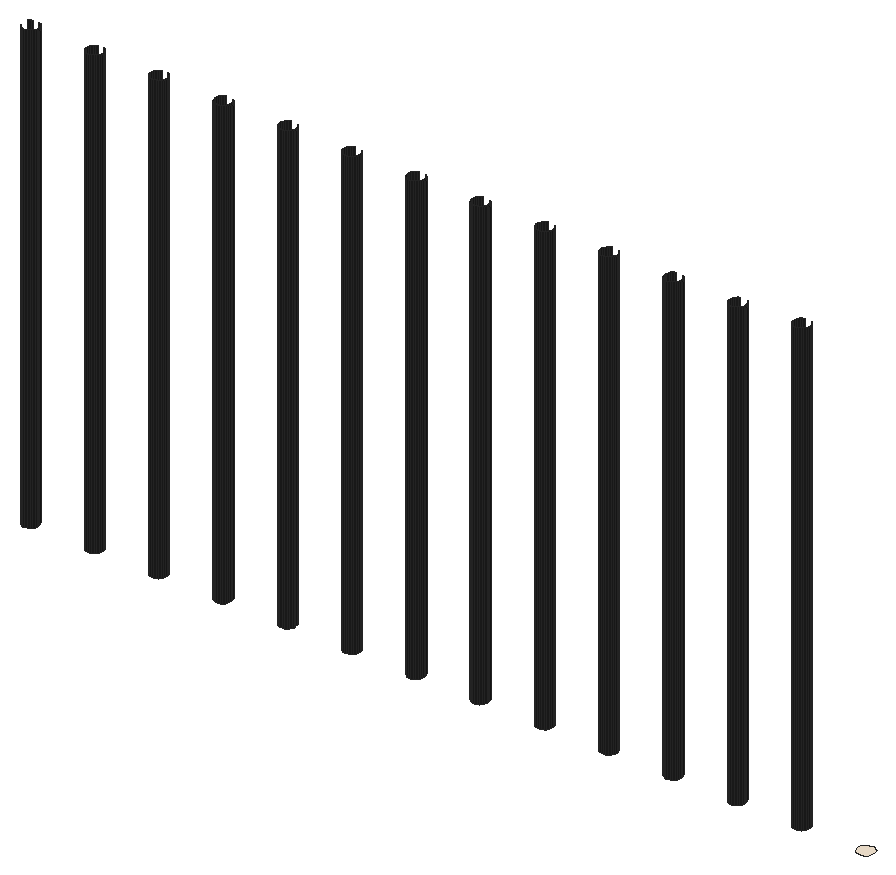
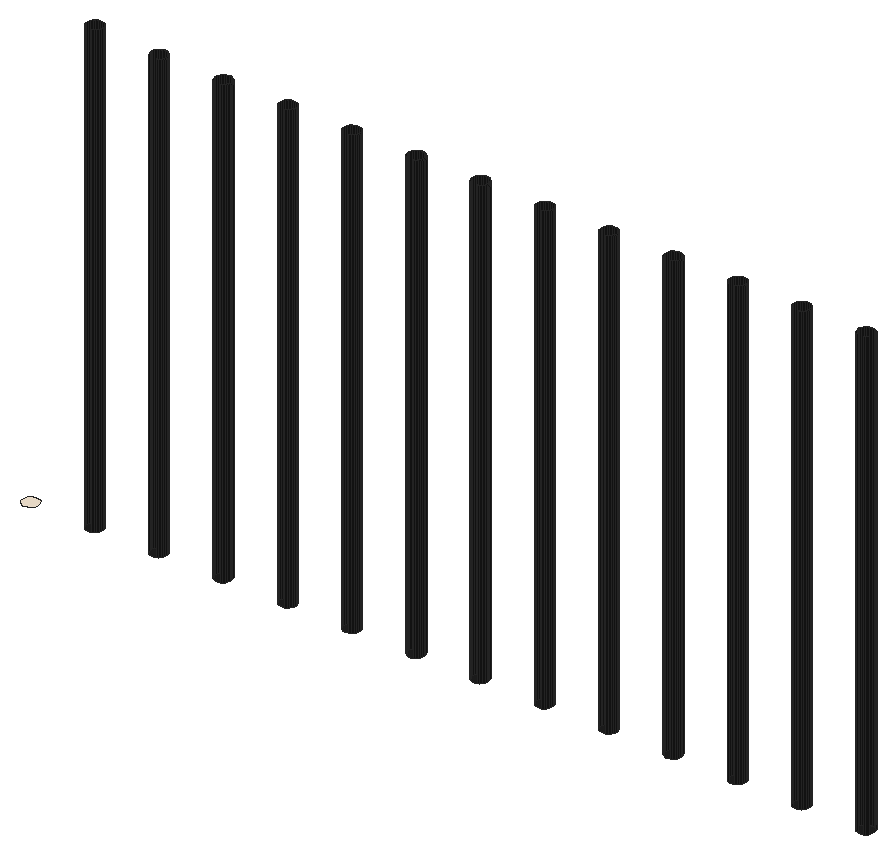
# SketchUp Ruby script. Lengths in inches.
U = 1.inch
M = Sketchup.active_model
def pt(a) = Geom::Point3d.new(a.map { |v| v * U })
def face(e, loops, mat)
  f = e.add_face(loops[0].map { |a| pt(a) })
  loops[1..].each { |l| e.add_face(l.map { |a| pt(a) }).erase! }
  f.material = f.back_material = mat if mat
  f
end
# faces: each face lists its corners as indices into pts; further lists are holes
def faces(e, pts, list, mat = nil) = list.each { |f| face(e, (f[0].is_a?(Array) ? f : [f]).map { |l| l.map { |i| pts[i] } }, mat) }
# xy, xz, yz: faces in a plane at the given z, y or x. An outline is a flat list of corners, or four numbers for a rectangle; further outlines are holes
def ring(l) = l.size == 4 ? [[l[0], l[1]], [l[2], l[1]], [l[2], l[3]], [l[0], l[3]]] : l.each_slice(2).to_a
def flat(e, list, mat, &to3) = list.each { |f| face(e, (f[0].is_a?(Array) ? f : [f]).map { |l| ring(l).map { |u, v| to3.(u, v) } }, mat) }
def xy(e, z, list, mat = nil) = flat(e, list, mat) { |x, y| [x, y, z] }
def xz(e, y, list, mat = nil) = flat(e, list, mat) { |x, z| [x, y, z] }
def yz(e, x, list, mat = nil) = flat(e, list, mat) { |y, z| [x, y, z] }
def lines(e, pts, list) = list.each { |a, b| e.add_line(pt(pts[a]), pt(pts[b])) }
# prism: a flat outline (further loops are holes) pulled along v
def prism(e, loops, v, mat = nil)
  f = face(e, loops, mat); d = Geom::Vector3d.new(v.map { |x| x * U })
  f.pushpull(f.normal.samedirection?(d) ? d.length : -d.length)
end
def box(e, o, s, mat = nil) = prism(e, [[o, [o[0] + s[0], o[1], o[2]], [o[0] + s[0], o[1] + s[1], o[2]], [o[0], o[1] + s[1], o[2]]]], [0, 0, s[2]], mat)
def at(x, y, z, deg = 0) = Geom::Transformation.translation(pt([x, y, z])) * Geom::Transformation.rotation(ORIGIN, Z_AXIS, deg.degrees)
def axes(o, x, y, z) = Geom::Transformation.new([*x, 0, *y, 0, *z, 0, *pt(o).to_a, 1])
def part(name) = M.definitions.add(name)
# library, detail: a bought-in or finely detailed component or shape, given as its bounding box
def library(name, o, s) = part(name).tap { |d| box(d.entities, o, s) }
def detail(e, o, s) = box(e.add_group.entities, o, s)
def put(e, d, t, mat = nil) = e.add_instance(d, t).tap { |i| i.material = mat if mat }
def group(e, t, mat = nil) = e.add_group.tap { |g| g.transformation = t; g.material = mat if mat }.entities
root = M.entities
M.materials.add("[0028_AntiqueWhite]").color = [250, 235, 215]
M.materials.add("[Color M08]").color = [30, 30, 30]
xy(root,177,[[209.92,194.68,210.0625,194.68,210.21,194.72,210.33,194.79,210.4375,194.89,210.51,195.02,210.55,195.16,210.55,195.31,210.51,195.45,210.44,195.58,210.33,195.68,210.2,195.75,210.0625,195.79,209.92,195.79,209.77,195.75,209.65,195.68,209.54,195.58,209.47,195.45,209.43,195.31,209.43,195.16,209.47,195.02,209.54,194.89,209.65,194.79,209.78,194.71]],"[0028_AntiqueWhite]")
xy(root,177,[[150.6,194.68,150.46,194.71,150.34,194.79,150.23,194.89,150.16,195.02,150.12,195.16,150.12,195.31,150.16,195.45,150.23,195.58,150.33,195.68,150.46,195.75,150.6,195.79,150.75,195.79,150.89,195.75,151.02,195.68,151.12,195.58,151.2,195.45,151.23,195.31,151.24,195.16,151.2,195.02,151.125,194.89,151.02,194.79,150.89,194.72,150.75,194.68],[155.17,194.68,155.03,194.71,154.9,194.79,154.79,194.89,154.72,195.02,154.68,195.16,154.68,195.31,154.72,195.45,154.79,195.58,154.9,195.68,155.02,195.75,155.17,195.79,155.3125,195.79,155.45,195.75,155.58,195.68,155.69,195.58,155.76,195.45,155.8,195.31,155.8,195.16,155.76,195.02,155.6875,194.89,155.58,194.79,155.46,194.72,155.3125,194.68],[159.73,194.68,159.59,194.71,159.46,194.79,159.36,194.89,159.28,195.02,159.24,195.16,159.24,195.31,159.28,195.45,159.36,195.58,159.46,195.68,159.59,195.75,159.73,195.79,159.875,195.79,160.02,195.75,160.14,195.68,160.25,195.58,160.32,195.45,160.36,195.31,160.36,195.16,160.32,195.02,160.25,194.89,160.15,194.79,160.02,194.72,159.875,194.68],[164.29,194.68,164.15,194.71,164.02,194.79,163.92,194.89,163.85,195.02,163.81,195.16,163.81,195.31,163.84,195.45,163.92,195.58,164.02,195.68,164.15,195.75,164.29,195.79,164.4375,195.79,164.58,195.75,164.71,195.68,164.81,195.58,164.88,195.45,164.92,195.31,164.92,195.16,164.88,195.02,164.8125,194.89,164.71,194.79,164.58,194.72,164.4375,194.68],[168.85,194.68,168.71,194.71,168.59,194.79,168.48,194.89,168.41,195.02,168.37,195.16,168.37,195.31,168.41,195.45,168.48,195.58,168.58,195.68,168.71,195.75,168.85,195.79,169,195.79,169.14,195.75,169.27,195.68,169.37,195.58,169.45,195.45,169.48,195.31,169.49,195.16,169.45,195.02,169.375,194.89,169.27,194.79,169.14,194.72,169,194.68],
  [173.42,194.68,173.28,194.71,173.15,194.79,173.04,194.89,172.97,195.02,172.93,195.16,172.93,195.31,172.97,195.45,173.04,195.58,173.15,195.68,173.27,195.75,173.42,195.79,173.5625,195.79,173.7,195.75,173.83,195.68,173.94,195.58,174.01,195.45,174.05,195.31,174.05,195.16,174.01,195.02,173.9375,194.89,173.83,194.79,173.71,194.72,173.5625,194.68],[177.98,194.68,177.84,194.71,177.71,194.79,177.61,194.89,177.53,195.02,177.49,195.16,177.49,195.31,177.53,195.45,177.61,195.58,177.71,195.68,177.84,195.75,177.98,195.79,178.125,195.79,178.27,195.75,178.39,195.68,178.5,195.58,178.57,195.45,178.61,195.31,178.61,195.16,178.57,195.02,178.5,194.89,178.4,194.79,178.27,194.72,178.125,194.68],[182.54,194.68,182.4,194.71,182.27,194.79,182.17,194.89,182.1,195.02,182.06,195.16,182.06,195.31,182.09,195.45,182.17,195.58,182.27,195.68,182.4,195.75,182.54,195.79,182.6875,195.79,182.83,195.75,182.96,195.68,183.06,195.58,183.13,195.45,183.17,195.31,183.17,195.16,183.13,195.02,183.0625,194.89,182.96,194.79,182.83,194.72,182.6875,194.68],[187.1,194.68,186.96,194.71,186.84,194.79,186.73,194.89,186.66,195.02,186.62,195.16,186.62,195.31,186.66,195.45,186.73,195.58,186.83,195.68,186.96,195.75,187.1,195.79,187.25,195.79,187.39,195.75,187.52,195.68,187.62,195.58,187.7,195.45,187.73,195.31,187.74,195.16,187.7,195.02,187.625,194.89,187.52,194.79,187.39,194.72,187.25,194.68],[191.67,194.68,191.53,194.71,191.4,194.79,191.29,194.89,191.22,195.02,191.18,195.16,191.18,195.31,191.22,195.45,191.29,195.58,191.4,195.68,191.52,195.75,191.67,195.79,191.8125,195.79,191.95,195.75,192.08,195.68,192.19,195.58,192.26,195.45,192.3,195.31,192.3,195.16,192.26,195.02,192.1875,194.89,192.08,194.79,191.96,194.72,191.8125,194.68],
  [196.23,194.68,196.09,194.71,195.96,194.79,195.86,194.89,195.78,195.02,195.74,195.16,195.74,195.31,195.78,195.45,195.86,195.58,195.96,195.68,196.09,195.75,196.23,195.79,196.375,195.79,196.52,195.75,196.64,195.68,196.75,195.58,196.82,195.45,196.86,195.31,196.86,195.16,196.82,195.02,196.75,194.89,196.65,194.79,196.52,194.72,196.375,194.68],[200.79,194.68,200.65,194.71,200.52,194.79,200.42,194.89,200.35,195.02,200.31,195.16,200.31,195.31,200.34,195.45,200.42,195.58,200.52,195.68,200.65,195.75,200.79,195.79,200.9375,195.79,201.08,195.75,201.21,195.68,201.31,195.58,201.38,195.45,201.42,195.31,201.42,195.16,201.38,195.02,201.3125,194.89,201.21,194.79,201.08,194.72,200.9375,194.68],[205.35,194.68,205.21,194.71,205.09,194.79,204.98,194.89,204.91,195.02,204.87,195.16,204.87,195.31,204.91,195.45,204.98,195.58,205.08,195.68,205.21,195.75,205.35,195.79,205.5,195.79,205.64,195.75,205.77,195.68,205.87,195.58,205.95,195.45,205.98,195.31,205.99,195.16,205.95,195.02,205.875,194.89,205.77,194.79,205.64,194.72,205.5,194.68]],"[Color M08]")
xz(root,194.68,[[150.6,177,150.75,208.66],[155.17,177,155.3125,208.66],[159.73,177,159.875,208.66],[164.29,177,164.4375,208.66],[168.85,177,169,208.66],
  [173.42,177,173.5625,208.625],[177.98,177,178.125,208.66],[182.54,177,182.6875,208.66],[187.1,177,187.25,208.66],[191.67,177,191.8125,208.66],
  [196.23,177,196.375,208.66],[200.79,177,200.9375,208.66],[205.35,177,205.5,208.9375]],"[Color M08]")
yz(root,154.68,[[195.16,177,195.31,208.66]],"[Color M08]")
yz(root,155.8,[[195.16,177,195.31,208.66]],"[Color M08]")
yz(root,159.24,[[195.16,177,195.31,208.66]],"[Color M08]")
yz(root,160.36,[[195.16,177,195.31,208.66]],"[Color M08]")
yz(root,163.81,[[195.16,177,195.31,208.66]],"[Color M08]")
yz(root,164.92,[[195.16,177,195.31,208.66]],"[Color M08]")
yz(root,168.37,[[195.16,177,195.31,208.66]],"[Color M08]")
yz(root,172.93,[[195.16,177,195.31,208.625]],"[Color M08]")
yz(root,174.05,[[195.16,177,195.31,208.625]],"[Color M08]")
yz(root,177.49,[[195.16,177,195.31,208.66]],"[Color M08]")
yz(root,178.61,[[195.16,177,195.31,208.66]],"[Color M08]")
yz(root,182.06,[[195.16,177,195.31,208.66]],"[Color M08]")
yz(root,183.17,[[195.16,177,195.31,208.66]],"[Color M08]")
yz(root,186.62,[[195.16,177,195.31,208.66]],"[Color M08]")
yz(root,191.18,[[195.16,177,195.31,208.66]],"[Color M08]")
yz(root,192.3,[[195.16,177,195.31,208.66]],"[Color M08]")
yz(root,195.74,[[195.16,177,195.31,208.66]],"[Color M08]")
yz(root,196.86,[[195.16,177,195.31,208.66]],"[Color M08]")
yz(root,200.31,[[195.16,177,195.31,208.66]],"[Color M08]")
yz(root,201.42,[[195.16,177,195.31,208.66]],"[Color M08]")
yz(root,204.87,[[195.16,177,195.31,208.9375]],"[Color M08]")
p = [[150.34,194.79,177],[150.46,194.71,177],[150.46,194.71,208.66],[150.34,194.79,208.66],[150.6,194.68,177],[150.6,194.68,208.66],
  [150.75,194.68,177],[150.89,194.72,177],[150.89,194.72,208.66],[150.75,194.68,208.66],[151.02,194.79,177],[151.02,194.79,208.66],
  [154.9,194.79,177],[155.03,194.71,177],[155.03,194.71,208.66],[154.9,194.79,208.66],[155.17,194.68,177],[155.17,194.68,208.66],
  [155.3125,194.68,177],[155.46,194.72,177],[155.46,194.72,208.66],[155.3125,194.68,208.66],[155.58,194.79,177],[155.58,194.79,208.66],
  [159.46,194.79,177],[159.59,194.71,177],[159.59,194.71,208.66],[159.46,194.79,208.66],[159.73,194.68,177],[159.73,194.68,208.66],
  [159.875,194.68,177],[160.02,194.72,177],[160.02,194.72,208.66],[159.875,194.68,208.66],[160.15,194.79,177],[160.15,194.79,208.66],
  [164.02,194.79,177],[164.15,194.71,177],[164.15,194.71,208.66],[164.02,194.79,208.66],[164.29,194.68,177],[164.29,194.68,208.66],
  [164.4375,194.68,177],[164.58,194.72,177],[164.58,194.72,208.66],[164.4375,194.68,208.66],[164.71,194.79,177],[164.71,194.79,208.66],
  [168.59,194.79,177],[168.71,194.71,177],[168.71,194.71,208.66],[168.59,194.79,208.66],[168.85,194.68,177],[168.85,194.68,208.66],
  [169,194.68,177],[169.14,194.72,177],[169.14,194.72,208.66],[169,194.68,208.66],[169.27,194.79,177],[169.27,194.79,208.66],
  [173.15,194.79,177],[173.28,194.71,177],[173.28,194.71,208.625],[173.15,194.79,208.625],[173.42,194.68,177],[173.42,194.68,208.625],
  [173.5625,194.68,177],[173.71,194.72,177],[173.71,194.72,208.625],[173.5625,194.68,208.625],[173.83,194.79,177],[173.83,194.79,208.625],
  [177.71,194.79,177],[177.84,194.71,177],[177.84,194.71,208.66],[177.71,194.79,208.66],[177.98,194.68,177],[177.98,194.68,208.66],
  [178.125,194.68,177],[178.27,194.72,177],[178.27,194.72,208.66],[178.125,194.68,208.66],[178.4,194.79,177],[178.4,194.79,208.66],
  [182.27,194.79,177],[182.4,194.71,177],[182.4,194.71,208.66],[182.27,194.79,208.66],[182.54,194.68,177],[182.54,194.68,208.66],
  [182.6875,194.68,177],[182.83,194.72,177],[182.83,194.72,208.66],[182.6875,194.68,208.66],[182.96,194.79,177],[182.96,194.79,208.66],
  [186.84,194.79,177],[186.96,194.71,177],[186.96,194.71,208.66],[186.84,194.79,208.66],[187.1,194.68,177],[187.1,194.68,208.66],
  [187.25,194.68,177],[187.39,194.72,177],[187.39,194.72,208.66],[187.25,194.68,208.66],[187.52,194.79,177],[187.52,194.79,208.66],
  [191.4,194.79,177],[191.53,194.71,177],[191.53,194.71,208.66],[191.4,194.79,208.66],[191.67,194.68,177],[191.67,194.68,208.66],
  [191.8125,194.68,177],[191.96,194.72,177],[191.96,194.72,208.66],[191.8125,194.68,208.66],[192.08,194.79,177],[192.08,194.79,208.66],
  [195.96,194.79,177],[196.09,194.71,177],[196.09,194.71,208.66],[195.96,194.79,208.66],[196.23,194.68,177],[196.23,194.68,208.66],
  [196.375,194.68,177],[196.52,194.72,177],[196.52,194.72,208.66],[196.375,194.68,208.66],[196.65,194.79,177],[196.65,194.79,208.66],
  [200.52,194.79,177],[200.65,194.71,177],[200.65,194.71,208.66],[200.52,194.79,208.66],[200.79,194.68,177],[200.79,194.68,208.66],
  [200.9375,194.68,177],[201.08,194.72,177],[201.08,194.72,208.66],[200.9375,194.68,208.66],[201.21,194.79,177],[201.21,194.79,208.66],
  [205.09,194.79,177],[205.21,194.71,177],[205.21,194.71,208.9375],[205.09,194.79,208.9375],[205.35,194.68,177],[205.35,194.68,208.9375],
  [205.5,194.68,177],[205.64,194.72,177],[205.64,194.72,208.9375],[205.5,194.68,208.9375],[205.77,194.79,177],[205.77,194.79,208.9375],
  [150.23,194.89,177],[150.23,194.89,208.66],[151.125,194.89,177],[151.125,194.89,208.66],[154.79,194.89,177],[154.79,194.89,208.66],
  [155.6875,194.89,177],[155.6875,194.89,208.66],[159.36,194.89,177],[159.36,194.89,208.66],[160.25,194.89,177],[160.25,194.89,208.66],
  [163.92,194.89,177],[163.92,194.89,208.66],[164.8125,194.89,177],[164.8125,194.89,208.66],[168.48,194.89,177],[168.48,194.89,208.66],
  [169.375,194.89,177],[169.375,194.89,208.66],[173.04,194.89,177],[173.04,194.89,208.625],[173.9375,194.89,177],[173.9375,194.89,208.625],
  [177.61,194.89,177],[177.61,194.89,208.66],[178.5,194.89,177],[178.5,194.89,208.66],[182.17,194.89,177],[182.17,194.89,208.66],
  [183.0625,194.89,177],[183.0625,194.89,208.66],[186.73,194.89,177],[186.73,194.89,208.66],[187.625,194.89,177],[187.625,194.89,208.66],
  [191.29,194.89,177],[191.29,194.89,208.66],[192.1875,194.89,177],[192.1875,194.89,208.66],[195.86,194.89,177],[195.86,194.89,208.66],
  [196.75,194.89,177],[196.75,194.89,208.66],[200.42,194.89,177],[200.42,194.89,208.66],[201.3125,194.89,177],[201.3125,194.89,208.66],
  [204.98,194.89,177],[204.98,194.89,208.9375],[205.875,194.89,177],[205.875,194.89,208.9375],[151.2,195.02,177],[151.2,195.02,208.66],
  [154.72,195.02,177],[154.72,195.02,208.66],[155.76,195.02,177],[155.76,195.02,208.66],[159.28,195.02,177],[159.28,195.02,208.66],
  [160.32,195.02,177],[160.32,195.02,208.66],[163.85,195.02,177],[163.85,195.02,208.66],[164.88,195.02,177],[164.88,195.02,208.66],
  [168.41,195.02,177],[168.41,195.02,208.66],[169.45,195.02,177],[169.45,195.02,208.66],[172.97,195.02,177],[172.97,195.02,208.625],
  [174.01,195.02,177],[174.01,195.02,208.625],[177.53,195.02,177],[177.53,195.02,208.66],[178.57,195.02,177],[178.57,195.02,208.66],
  [182.1,195.02,177],[182.1,195.02,208.66],[183.13,195.02,177],[183.13,195.02,208.66],[186.66,195.02,177],[186.66,195.02,208.66],
  [187.7,195.02,177],[187.7,195.02,208.66],[191.22,195.02,177],[191.22,195.02,208.66],[192.26,195.02,177],[192.26,195.02,208.66],
  [195.78,195.02,177],[195.78,195.02,208.66],[196.82,195.02,177],[196.82,195.02,208.66],[200.35,195.02,177],[200.35,195.02,208.66],
  [201.38,195.02,177],[201.38,195.02,208.66],[204.91,195.02,177],[204.91,195.02,208.9375],[205.95,195.02,177],[205.95,195.02,208.9375],
  [151.24,195.16,177],[151.24,195.16,208.66],[154.68,195.16,177],[154.68,195.16,208.66],[155.8,195.16,177],[155.8,195.16,208.66],
  [159.24,195.16,177],[159.24,195.16,208.66],[160.36,195.16,177],[160.36,195.16,208.66],[163.81,195.16,177],[163.81,195.16,208.66],
  [164.92,195.16,177],[164.92,195.16,208.66],[168.37,195.16,177],[168.37,195.16,208.66],[169.49,195.16,177],[169.49,195.16,208.66],
  [172.93,195.16,177],[172.93,195.16,208.625],[174.05,195.16,177],[174.05,195.16,208.625],[177.49,195.16,177],[177.49,195.16,208.66],
  [178.61,195.16,177],[178.61,195.16,208.66],[182.06,195.16,177],[182.06,195.16,208.66],[183.17,195.16,177],[183.17,195.16,208.66],
  [186.62,195.16,177],[186.62,195.16,208.66],[187.74,195.16,177],[187.74,195.16,208.66],[191.18,195.16,177],[191.18,195.16,208.66],
  [192.3,195.16,177],[192.3,195.16,208.66],[195.74,195.16,177],[195.74,195.16,208.66],[196.86,195.16,177],[196.86,195.16,208.66],
  [200.31,195.16,177],[200.31,195.16,208.66],[201.42,195.16,177],[201.42,195.16,208.66],[204.87,195.16,177],[204.87,195.16,208.9375],
  [205.99,195.16,177],[205.99,195.16,208.9375],[151.23,195.31,177],[151.23,195.31,208.66],[169.48,195.31,177],[169.48,195.31,208.66],
  [187.73,195.31,177],[187.73,195.31,208.66],[205.98,195.31,177],[205.98,195.31,208.9375],[151.2,195.45,177],[151.2,195.45,208.66],
  [154.72,195.45,177],[154.68,195.31,177],[154.68,195.31,208.66],[154.72,195.45,208.66],[155.8,195.31,177],[155.76,195.45,177],
  [155.76,195.45,208.66],[155.8,195.31,208.66],[159.28,195.45,177],[159.24,195.31,177],[159.24,195.31,208.66],[159.28,195.45,208.66],
  [160.36,195.31,177],[160.32,195.45,177],[160.32,195.45,208.66],[160.36,195.31,208.66],[163.84,195.45,177],[163.81,195.31,177],
  [163.81,195.31,208.66],[163.84,195.45,208.66],[164.92,195.31,177],[164.88,195.45,177],[164.88,195.45,208.66],[164.92,195.31,208.66],
  [168.41,195.45,177],[168.37,195.31,177],[168.37,195.31,208.66],[168.41,195.45,208.66],[169.45,195.45,177],[169.45,195.45,208.66],
  [172.97,195.45,177],[172.93,195.31,177],[172.93,195.31,208.625],[172.97,195.45,208.625],[174.05,195.31,177],[174.01,195.45,177],
  [174.01,195.45,208.625],[174.05,195.31,208.625],[177.53,195.45,177],[177.49,195.31,177],[177.49,195.31,208.66],[177.53,195.45,208.66],
  [178.61,195.31,177],[178.57,195.45,177],[178.57,195.45,208.66],[178.61,195.31,208.66],[182.09,195.45,177],[182.06,195.31,177],
  [182.06,195.31,208.66],[182.09,195.45,208.66],[183.17,195.31,177],[183.13,195.45,177],[183.13,195.45,208.66],[183.17,195.31,208.66],
  [186.66,195.45,177],[186.62,195.31,177],[186.62,195.31,208.66],[186.66,195.45,208.66],[187.7,195.45,177],[187.7,195.45,208.66],
  [191.22,195.45,177],[191.18,195.31,177],[191.18,195.31,208.66],[191.22,195.45,208.66],[192.3,195.31,177],[192.26,195.45,177],
  [192.26,195.45,208.66],[192.3,195.31,208.66],[195.78,195.45,177],[195.74,195.31,177],[195.74,195.31,208.66],[195.78,195.45,208.66],
  [196.86,195.31,177],[196.82,195.45,177],[196.82,195.45,208.66],[196.86,195.31,208.66],[200.34,195.45,177],[200.31,195.31,177],
  [200.31,195.31,208.66],[200.34,195.45,208.66],[201.42,195.31,177],[201.38,195.45,177],[201.38,195.45,208.66],[201.42,195.31,208.66],
  [204.91,195.45,177],[204.87,195.31,177],[204.87,195.31,208.9375],[204.91,195.45,208.9375],[205.95,195.45,177],[205.95,195.45,208.9375],
  [154.79,195.58,177],[154.79,195.58,208.66],[159.36,195.58,177],[159.36,195.58,208.66],[163.92,195.58,177],[163.92,195.58,208.66],
  [168.48,195.58,177],[168.48,195.58,208.66],[173.04,195.58,177],[173.04,195.58,208.625],[177.61,195.58,177],[177.61,195.58,208.66],
  [182.17,195.58,177],[182.17,195.58,208.66],[186.73,195.58,177],[186.73,195.58,208.66],[191.29,195.58,177],[191.29,195.58,208.66],
  [195.86,195.58,177],[195.86,195.58,208.66],[200.42,195.58,177],[200.42,195.58,208.66],[204.98,195.58,177],[204.98,195.58,208.9375],
  [151.12,195.58,177],[151.12,195.58,208.66],[155.69,195.58,177],[155.69,195.58,208.66],[160.25,195.58,177],[160.25,195.58,208.66],
  [164.81,195.58,177],[164.81,195.58,208.66],[169.37,195.58,177],[169.37,195.58,208.66],[173.94,195.58,177],[173.94,195.58,208.625],
  [178.5,195.58,177],[178.5,195.58,208.66],[183.06,195.58,177],[183.06,195.58,208.66],[187.62,195.58,177],[187.62,195.58,208.66],
  [192.19,195.58,177],[192.19,195.58,208.66],[196.75,195.58,177],[196.75,195.58,208.66],[201.31,195.58,177],[201.31,195.58,208.66],
  [205.87,195.58,177],[205.87,195.58,208.9375],[150.33,195.68,177],[150.23,195.58,177],[150.23,195.58,208.66],[150.33,195.68,208.66],
  [151.02,195.68,177],[151.02,195.68,208.66],[154.9,195.68,177],[154.9,195.68,208.66],[155.58,195.68,177],[155.58,195.68,208.66],
  [159.46,195.68,177],[159.46,195.68,208.66],[160.14,195.68,177],[160.14,195.68,208.66],[164.02,195.68,177],[164.02,195.68,208.66],
  [164.71,195.68,177],[164.71,195.68,208.66],[168.58,195.68,177],[168.58,195.68,208.66],[169.27,195.68,177],[169.27,195.68,208.66],
  [173.15,195.68,177],[173.15,195.68,208.625],[173.83,195.68,177],[173.83,195.68,208.625],[177.71,195.68,177],[177.71,195.68,208.66],
  [178.39,195.68,177],[178.39,195.68,208.66],[182.27,195.68,177],[182.27,195.68,208.66],[182.96,195.68,177],[182.96,195.68,208.66],
  [186.83,195.68,177],[186.83,195.68,208.66],[187.52,195.68,177],[187.52,195.68,208.66],[191.4,195.68,177],[191.4,195.68,208.66],
  [192.08,195.68,177],[192.08,195.68,208.66],[195.96,195.68,177],[195.96,195.68,208.66],[196.64,195.68,177],[196.64,195.68,208.66],
  [200.52,195.68,177],[200.52,195.68,208.66],[201.21,195.68,177],[201.21,195.68,208.66],[205.08,195.68,177],[205.08,195.68,208.9375],
  [205.77,195.68,177],[205.77,195.68,208.9375],[150.46,195.75,177],[150.46,195.75,208.66],[150.89,195.75,177],[150.89,195.75,208.66],
  [155.02,195.75,177],[155.02,195.75,208.66],[155.45,195.75,177],[155.45,195.75,208.66],[159.59,195.75,177],[159.59,195.75,208.66],
  [160.02,195.75,177],[160.02,195.75,208.66],[164.15,195.75,177],[164.15,195.75,208.66],[168.71,195.75,177],[168.71,195.75,208.66],
  [173.27,195.75,177],[173.27,195.75,208.625],[177.84,195.75,177],[177.84,195.75,208.66],[182.4,195.75,177],[182.4,195.75,208.66],
  [186.96,195.75,177],[186.96,195.75,208.66],[191.52,195.75,177],[191.52,195.75,208.66],[196.09,195.75,177],[196.09,195.75,208.66],
  [200.65,195.75,177],[200.65,195.75,208.66],[205.21,195.75,177],[205.21,195.75,208.9375]]
faces(root,p,[[0,1,2,3],[1,4,5,2],[6,7,8,9],[7,10,11,8],[12,13,14,15],[13,16,17,14],[18,19,20,21],[19,22,23,20],
  [24,25,26,27],[25,28,29,26],[30,31,32,33],[31,34,35,32],[36,37,38,39],[37,40,41,38],[42,43,44,45],[43,46,47,44],
  [48,49,50,51],[49,52,53,50],[54,55,56,57],[55,58,59,56],[60,61,62,63],[61,64,65,62],[66,67,68,69],[67,70,71,68],
  [72,73,74,75],[73,76,77,74],[78,79,80,81],[79,82,83,80],[84,85,86,87],[85,88,89,86],[90,91,92,93],[91,94,95,92],
  [96,97,98,99],[97,100,101,98],[102,103,104,105],[103,106,107,104],[108,109,110,111],[109,112,113,110],[114,115,116,117],[115,118,119,116],
  [120,121,122,123],[121,124,125,122],[126,127,128,129],[127,130,131,128],[132,133,134,135],[133,136,137,134],[138,139,140,141],[139,142,143,140],
  [144,145,146,147],[145,148,149,146],[150,151,152,153],[151,154,155,152],[156,0,3,157],[10,158,159,11],[160,12,15,161],[22,162,163,23],
  [164,24,27,165],[34,166,167,35],[168,36,39,169],[46,170,171,47],[172,48,51,173],[58,174,175,59],[176,60,63,177],[70,178,179,71],
  [180,72,75,181],[82,182,183,83],[184,84,87,185],[94,186,187,95],[188,96,99,189],[106,190,191,107],[192,108,111,193],[118,194,195,119],
  [196,120,123,197],[130,198,199,131],[200,132,135,201],[142,202,203,143],[204,144,147,205],[154,206,207,155],[158,208,209,159],[210,160,161,211],
  [162,212,213,163],[214,164,165,215],[166,216,217,167],[218,168,169,219],[170,220,221,171],[222,172,173,223],[174,224,225,175],[226,176,177,227],
  [178,228,229,179],[230,180,181,231],[182,232,233,183],[234,184,185,235],[186,236,237,187],[238,188,189,239],[190,240,241,191],[242,192,193,243],
  [194,244,245,195],[246,196,197,247],[198,248,249,199],[250,200,201,251],[202,252,253,203],[254,204,205,255],[206,256,257,207],[208,258,259,209],
  [260,210,211,261],[212,262,263,213],[264,214,215,265],[216,266,267,217],[268,218,219,269],[220,270,271,221],[272,222,223,273],[224,274,275,225],
  [276,226,227,277],[228,278,279,229],[280,230,231,281],[232,282,283,233],[284,234,235,285],[236,286,287,237],[288,238,239,289],[240,290,291,241],
  [292,242,243,293],[244,294,295,245],[296,246,247,297],[248,298,299,249],[300,250,251,301],[252,302,303,253],[304,254,255,305],[256,306,307,257],
  [258,308,309,259],[274,310,311,275],[290,312,313,291],[306,314,315,307],[308,316,317,309],[318,319,320,321],[322,323,324,325],[326,327,328,329],
  [330,331,332,333],[334,335,336,337],[338,339,340,341],[342,343,344,345],[310,346,347,311],[348,349,350,351],[352,353,354,355],[356,357,358,359],
  [360,361,362,363],[364,365,366,367],[368,369,370,371],[372,373,374,375],[312,376,377,313],[378,379,380,381],[382,383,384,385],[386,387,388,389],
  [390,391,392,393],[394,395,396,397],[398,399,400,401],[402,403,404,405],[314,406,407,315],[408,318,321,409],[410,326,329,411],[412,334,337,413],
  [414,342,345,415],[416,348,351,417],[418,356,359,419],[420,364,367,421],[422,372,375,423],[424,378,381,425],[426,386,389,427],[428,394,397,429],
  [430,402,405,431],[316,432,433,317],[323,434,435,324],[331,436,437,332],[339,438,439,340],[346,440,441,347],[353,442,443,354],[361,444,445,362],
  [369,446,447,370],[376,448,449,377],[383,450,451,384],[391,452,453,392],[399,454,455,400],[406,456,457,407],[458,459,460,461],[432,462,463,433],
  [464,408,409,465],[434,466,467,435],[468,410,411,469],[436,470,471,437],[472,412,413,473],[438,474,475,439],[476,414,415,477],[440,478,479,441],
  [480,416,417,481],[442,482,483,443],[484,418,419,485],[444,486,487,445],[488,420,421,489],[446,490,491,447],[492,422,423,493],[448,494,495,449],
  [496,424,425,497],[450,498,499,451],[500,426,427,501],[452,502,503,453],[504,428,429,505],[454,506,507,455],[508,430,431,509],[456,510,511,457],
  [512,458,461,513],[462,514,515,463],[516,464,465,517],[466,518,519,467],[520,468,469,521],[470,522,523,471],[524,472,473,525],[526,476,477,527],
  [528,480,481,529],[530,484,485,531],[532,488,489,533],[534,492,493,535],[536,496,497,537],[538,500,501,539],[540,504,505,541],[542,508,509,543]],"[Color M08]")
